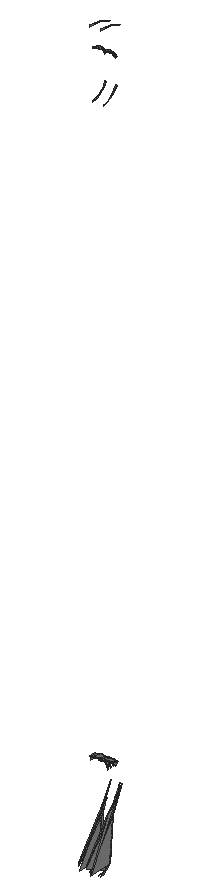
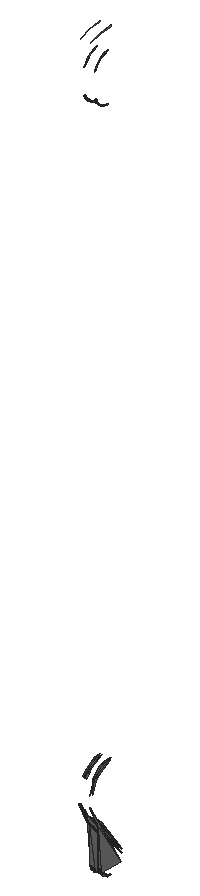
# SketchUp Ruby script. Lengths in inches.
U = 1.inch
M = Sketchup.active_model
def pt(a) = Geom::Point3d.new(a.map { |v| v * U })
def face(e, loops, mat)
  f = e.add_face(loops[0].map { |a| pt(a) })
  loops[1..].each { |l| e.add_face(l.map { |a| pt(a) }).erase! }
  f.material = f.back_material = mat if mat
  f
end
# faces: each face lists its corners as indices into pts; further lists are holes
def faces(e, pts, list, mat = nil) = list.each { |f| face(e, (f[0].is_a?(Array) ? f : [f]).map { |l| l.map { |i| pts[i] } }, mat) }
# xy, xz, yz: faces in a plane at the given z, y or x. An outline is a flat list of corners, or four numbers for a rectangle; further outlines are holes
def ring(l) = l.size == 4 ? [[l[0], l[1]], [l[2], l[1]], [l[2], l[3]], [l[0], l[3]]] : l.each_slice(2).to_a
def flat(e, list, mat, &to3) = list.each { |f| face(e, (f[0].is_a?(Array) ? f : [f]).map { |l| ring(l).map { |u, v| to3.(u, v) } }, mat) }
def xy(e, z, list, mat = nil) = flat(e, list, mat) { |x, y| [x, y, z] }
def xz(e, y, list, mat = nil) = flat(e, list, mat) { |x, z| [x, y, z] }
def yz(e, x, list, mat = nil) = flat(e, list, mat) { |y, z| [x, y, z] }
def lines(e, pts, list) = list.each { |a, b| e.add_line(pt(pts[a]), pt(pts[b])) }
# prism: a flat outline (further loops are holes) pulled along v
def prism(e, loops, v, mat = nil)
  f = face(e, loops, mat); d = Geom::Vector3d.new(v.map { |x| x * U })
  f.pushpull(f.normal.samedirection?(d) ? d.length : -d.length)
end
def box(e, o, s, mat = nil) = prism(e, [[o, [o[0] + s[0], o[1], o[2]], [o[0] + s[0], o[1] + s[1], o[2]], [o[0], o[1] + s[1], o[2]]]], [0, 0, s[2]], mat)
def at(x, y, z, deg = 0) = Geom::Transformation.translation(pt([x, y, z])) * Geom::Transformation.rotation(ORIGIN, Z_AXIS, deg.degrees)
def axes(o, x, y, z) = Geom::Transformation.new([*x, 0, *y, 0, *z, 0, *pt(o).to_a, 1])
def part(name) = M.definitions.add(name)
# library, detail: a bought-in or finely detailed component or shape, given as its bounding box
def library(name, o, s) = part(name).tap { |d| box(d.entities, o, s) }
def detail(e, o, s) = box(e.add_group.entities, o, s)
def put(e, d, t, mat = nil) = e.add_instance(d, t).tap { |i| i.material = mat if mat }
def group(e, t, mat = nil) = e.add_group.tap { |g| g.transformation = t; g.material = mat if mat }.entities
root = M.entities
M.materials.add("Material \#1").color = [140, 140, 140]
yz(root,362.564,[[201.798,46.486,201.837,46.491,201.873,46.505],[201.798,46.486,201.873,46.505,201.932,46.557],[201.873,46.505,201.905,46.528,201.932,46.557],[201.664,46.557,201.932,46.557,201.97,47.04],[201.664,46.557,201.976,47.061,202.103,47.295],
  [201.664,46.557,202.103,47.295,202.01,47.155],[201.932,46.557,201.952,46.591,201.965,46.631],[201.932,46.557,201.965,46.631,201.97,47.032],[201.932,46.557,201.97,47.032,201.97,47.04],[201.965,46.631,201.97,46.674,201.97,47.032],
  [201.976,47.061,201.98,47.067,202.103,47.295],[201.985,47.073,201.991,47.079,202.044,47.139],[201.991,47.079,202.019,47.107,202.044,47.139],[202.062,47.407,202.038,47.549,202.042,47.47],[202.097,47.416,202.074,47.487,202.038,47.549],
  [202.042,47.47,202.038,47.549,202.01,47.525],[202.01,47.525,202.038,47.549,201.968,47.57],[202.038,47.549,201.798,47.675,201.917,47.605],[202.038,47.549,201.933,47.641,201.798,47.675],[202.038,47.549,201.917,47.605,201.968,47.57],
  [202.038,47.549,201.99,47.601,201.933,47.641],[201.917,47.605,201.798,47.675,201.86,47.628],[201.933,47.641,201.868,47.666,201.798,47.675]],"Material \#1")
yz(root,362.566,[[201.845,54.307,201.889,54.32,201.842,54.321],[201.889,54.32,201.885,54.334,201.842,54.321],[201.889,54.32,201.93,54.341,201.885,54.334],[201.885,54.334,201.93,54.341,201.924,54.354],[201.93,54.341,201.967,54.369,201.924,54.354],
  [201.924,54.354,201.967,54.369,201.958,54.381],[201.967,54.369,201.999,54.404,201.958,54.381],[201.958,54.381,201.999,54.404,201.988,54.413],[201.999,54.404,202.025,54.444,201.988,54.413],[201.988,54.413,202.025,54.444,202.013,54.451],
  [202.013,54.726,201.999,54.773,201.988,54.764],[202.013,54.726,202.025,54.733,201.999,54.773],[201.988,54.764,201.967,54.808,201.958,54.796],[201.988,54.764,201.999,54.773,201.967,54.808],[201.958,54.796,201.93,54.836,201.924,54.823],
  [201.958,54.796,201.967,54.808,201.93,54.836],[201.924,54.823,201.889,54.857,201.885,54.843],[201.924,54.823,201.93,54.836,201.889,54.857],[201.885,54.843,201.845,54.87,201.842,54.856],[201.885,54.843,201.889,54.857,201.845,54.87],
  [202.069,55.038,201.94,55.092,201.9375,55.077],[201.9375,55.077,201.798,55.106,201.798,55.091],[201.9375,55.077,201.94,55.092,201.798,55.106]],"Material \#1")
yz(root,362.585,[[201.798,46.486,201.873,46.505,201.837,46.491],[201.873,46.505,201.932,46.557,201.905,46.528],[201.873,46.505,201.965,46.631,201.932,46.557],[201.873,46.505,201.97,47.032,201.965,46.631],[201.932,46.557,201.965,46.631,201.952,46.591],
  [201.63,46.631,201.97,47.04,201.97,47.032],[201.63,46.631,201.971,47.047,201.97,47.04],[201.63,46.631,201.973,47.054,201.971,47.047],[201.63,46.631,201.976,47.061,201.973,47.054],[201.965,46.631,201.97,47.032,201.97,46.674],
  [201.626,46.674,201.917,47.074,201.968,47.109],[201.626,46.674,201.968,47.109,202.01,47.155],[201.626,46.674,202.01,47.155,201.976,47.061],[202.042,47.47,202.01,47.525,202.038,47.549],[202.01,47.525,201.968,47.57,202.038,47.549],
  [202.038,47.549,201.798,47.675,201.933,47.641],[202.038,47.549,201.917,47.605,201.798,47.675],[202.038,47.549,201.968,47.57,201.917,47.605],[202.038,47.549,201.933,47.641,201.99,47.601],[201.917,47.605,201.86,47.628,201.798,47.675],
  [201.86,47.628,201.798,47.635,201.798,47.675],[201.933,47.641,201.798,47.675,201.868,47.666]],"Material \#1")
yz(root,362.667,[[201.798,46.486,201.837,46.491,201.873,46.505],[201.873,46.505,201.97,47.032,201.63,46.631],[201.873,46.505,201.905,46.528,201.932,46.557],[201.873,46.505,201.932,46.557,201.965,46.631],[201.873,46.505,201.965,46.631,201.97,47.032],
  [201.932,46.557,201.952,46.591,201.965,46.631],[201.63,46.631,201.97,47.032,201.97,47.04],[201.63,46.631,201.97,47.04,201.971,47.047],[201.63,46.631,201.971,47.047,201.973,47.054],[201.63,46.631,201.973,47.054,201.976,47.061],
  [201.965,46.631,201.97,46.674,201.97,47.032],[201.626,46.674,201.968,47.109,201.917,47.074],[201.626,46.674,201.976,47.061,202.01,47.155],[201.626,46.674,202.01,47.155,201.968,47.109],[201.976,47.061,201.98,47.067,202.103,47.295],
  [201.976,47.061,202.042,47.209,202.01,47.155],[201.985,47.073,201.991,47.079,202.044,47.139],[201.991,47.079,202.019,47.107,202.044,47.139],[202.01,47.525,202.038,47.549,201.968,47.57],[202.038,47.549,201.798,47.675,201.917,47.605],
  [202.038,47.549,201.933,47.641,201.798,47.675],[202.038,47.549,201.917,47.605,201.968,47.57],[202.038,47.549,201.99,47.601,201.933,47.641],[201.917,47.605,201.798,47.675,201.86,47.628],[201.933,47.641,201.868,47.666,201.798,47.675]],"Material \#1")
yz(root,362.685,[[201.845,54.307,201.842,54.321,201.889,54.32],[201.889,54.32,201.842,54.321,201.885,54.334],[201.889,54.32,201.885,54.334,201.93,54.341],[201.885,54.334,201.924,54.354,201.93,54.341],[201.93,54.341,201.924,54.354,201.967,54.369],
  [201.924,54.354,201.958,54.381,201.967,54.369],[201.967,54.369,201.958,54.381,201.999,54.404],[201.958,54.381,201.988,54.413,201.999,54.404],[201.999,54.404,201.988,54.413,202.025,54.444],[201.988,54.413,202.013,54.451,202.025,54.444],
  [202.013,54.726,201.988,54.764,201.999,54.773],[202.013,54.726,201.999,54.773,202.025,54.733],[201.988,54.764,201.958,54.796,201.967,54.808],[201.988,54.764,201.967,54.808,201.999,54.773],[201.958,54.796,201.924,54.823,201.93,54.836],
  [201.958,54.796,201.93,54.836,201.967,54.808],[201.924,54.823,201.885,54.843,201.889,54.857],[201.924,54.823,201.889,54.857,201.93,54.836],[201.885,54.843,201.842,54.856,201.845,54.87],[201.885,54.843,201.845,54.87,201.889,54.857],
  [202.069,55.038,201.9375,55.077,201.94,55.092],[201.9375,55.077,201.798,55.091,201.798,55.106],[201.9375,55.077,201.798,55.106,201.94,55.092]],"Material \#1")
yz(root,362.6875,[[201.798,46.486,201.873,46.505,201.837,46.491],[201.798,46.486,201.932,46.557,201.873,46.505],[201.664,46.557,201.917,47.074,201.968,47.109],[201.664,46.557,201.968,47.109,202.01,47.155],[201.664,46.557,201.97,47.04,201.932,46.557],
  [201.664,46.557,201.971,47.047,201.97,47.04],[201.664,46.557,201.973,47.054,201.971,47.047],[201.664,46.557,201.976,47.061,201.973,47.054],[201.664,46.557,202.01,47.155,202.103,47.295],[201.664,46.557,202.103,47.295,201.976,47.061],
  [201.932,46.557,201.97,47.04,201.97,47.032],[201.976,47.061,202.103,47.295,201.98,47.067],[202.01,47.525,201.968,47.57,202.038,47.549],[202.038,47.549,201.798,47.675,201.933,47.641],[202.038,47.549,201.917,47.605,201.798,47.675],
  [202.038,47.549,201.968,47.57,201.917,47.605],[202.038,47.549,201.933,47.641,201.99,47.601],[201.917,47.605,201.86,47.628,201.798,47.675],[201.933,47.641,201.798,47.675,201.868,47.666]],"Material \#1")
